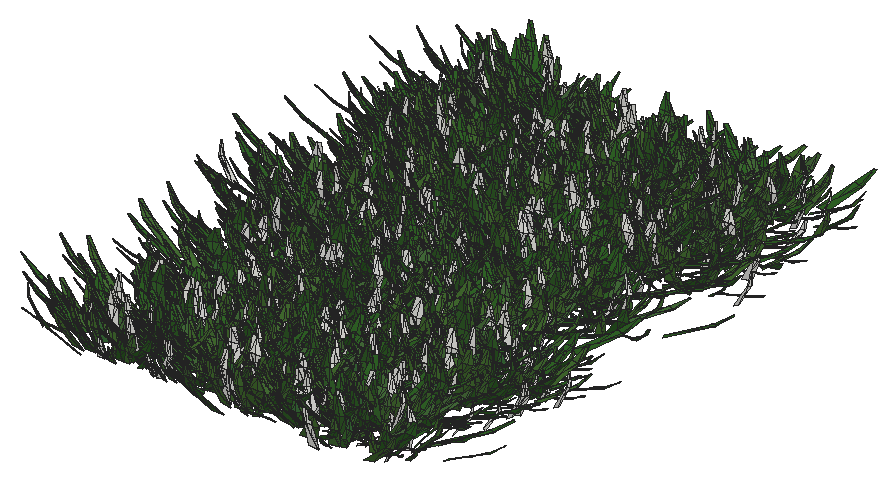
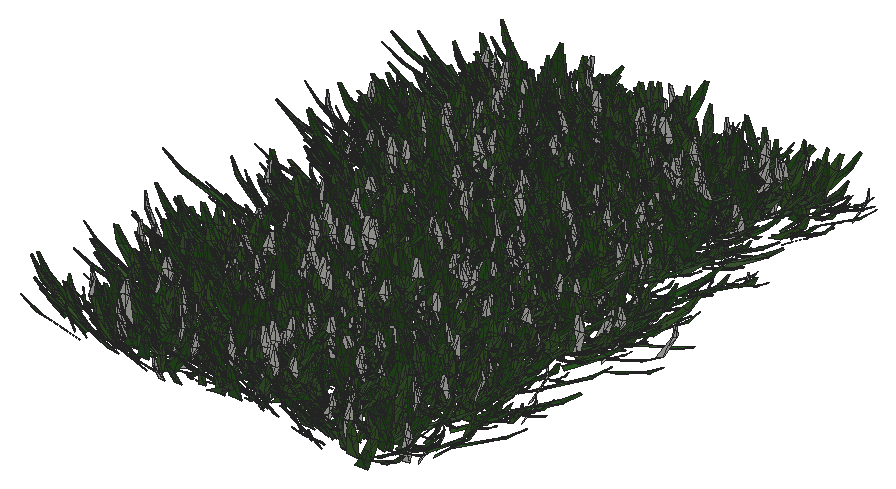
# SketchUp Ruby script. Lengths in inches.
U = 1.inch
M = Sketchup.active_model
def pt(a) = Geom::Point3d.new(a.map { |v| v * U })
def face(e, loops, mat)
  f = e.add_face(loops[0].map { |a| pt(a) })
  loops[1..].each { |l| e.add_face(l.map { |a| pt(a) }).erase! }
  f.material = f.back_material = mat if mat
  f
end
# faces: each face lists its corners as indices into pts; further lists are holes
def faces(e, pts, list, mat = nil) = list.each { |f| face(e, (f[0].is_a?(Array) ? f : [f]).map { |l| l.map { |i| pts[i] } }, mat) }
# xy, xz, yz: faces in a plane at the given z, y or x. An outline is a flat list of corners, or four numbers for a rectangle; further outlines are holes
def ring(l) = l.size == 4 ? [[l[0], l[1]], [l[2], l[1]], [l[2], l[3]], [l[0], l[3]]] : l.each_slice(2).to_a
def flat(e, list, mat, &to3) = list.each { |f| face(e, (f[0].is_a?(Array) ? f : [f]).map { |l| ring(l).map { |u, v| to3.(u, v) } }, mat) }
def xy(e, z, list, mat = nil) = flat(e, list, mat) { |x, y| [x, y, z] }
def xz(e, y, list, mat = nil) = flat(e, list, mat) { |x, z| [x, y, z] }
def yz(e, x, list, mat = nil) = flat(e, list, mat) { |y, z| [x, y, z] }
def lines(e, pts, list) = list.each { |a, b| e.add_line(pt(pts[a]), pt(pts[b])) }
# prism: a flat outline (further loops are holes) pulled along v
def prism(e, loops, v, mat = nil)
  f = face(e, loops, mat); d = Geom::Vector3d.new(v.map { |x| x * U })
  f.pushpull(f.normal.samedirection?(d) ? d.length : -d.length)
end
def box(e, o, s, mat = nil) = prism(e, [[o, [o[0] + s[0], o[1], o[2]], [o[0] + s[0], o[1] + s[1], o[2]], [o[0], o[1] + s[1], o[2]]]], [0, 0, s[2]], mat)
def at(x, y, z, deg = 0) = Geom::Transformation.translation(pt([x, y, z])) * Geom::Transformation.rotation(ORIGIN, Z_AXIS, deg.degrees)
def axes(o, x, y, z) = Geom::Transformation.new([*x, 0, *y, 0, *z, 0, *pt(o).to_a, 1])
def part(name) = M.definitions.add(name)
# library, detail: a bought-in or finely detailed component or shape, given as its bounding box
def library(name, o, s) = part(name).tap { |d| box(d.entities, o, s) }
def detail(e, o, s) = box(e.add_group.entities, o, s)
def put(e, d, t, mat = nil) = e.add_instance(d, t).tap { |i| i.material = mat if mat }
def group(e, t, mat = nil) = e.add_group.tap { |g| g.transformation = t; g.material = mat if mat }.entities
root = M.entities
M.materials.add("Material82").color = [68, 110, 58]
M.materials.add("Material83").color = [48, 90, 38]
M.materials.add("Material84").color = [68, 110, 48]
M.materials.add("Material85").color = [48, 90, 48]
M.materials.add("Material86").color = [58, 110, 58]
M.materials.add("Material87").color = [58, 90, 38]
M.materials.add("Material88").color = [68, 100, 58]
M.materials.add("Material89").color = [48, 100, 38]
c1 = part("grass00")
p = [[-0.6875,0.15,0],[-0.56,0.08,5.52],[-0.04,0.03,2.76],[0.48,-0.02,0],[0.35,-0.02,5.52],[-0.1,-0.14,5.52],
  [-0.12,0.65,8.37],[-0.42,0.65,8.37]]
faces(c1.entities,p,[[0,1,2,3],[3,2,4],[1,5,2],[5,4,2],[1,6,5],[4,5,6],[7,6,1]])
c2 = part("Group16\#1")
put(c2.entities,c1,axes([1.44,-0.61,-0.01],[0.05352,0.12609,0],[-0.10704,0.04543,0.07239],[0.06664,-0.02828,0.11628]),"Material85")
put(c2.entities,c1,axes([0.76,-0.15,-0.01],[0.04676,0.24062,0],[-0.23162,0.04501,0.06642],[0.0652,-0.01267,0.23595]),"Material82")
put(c2.entities,c1,axes([0.79,0.01,-0.01],[-0.00606,0.34651,0],[-0.34381,-0.00602,0.0432],[0.04319,0.00076,0.34386]))
put(c2.entities,c1,axes([1,0.23,-0.01],[-0.07192,0.31144,0],[-0.28722,-0.06632,0.1236],[0.12043,0.02781,0.29478]),"Material84")
put(c2.entities,c1,axes([1.66,0.77,-0.01],[-0.13828,0.29651,0],[-0.21551,-0.1005,0.22471],[0.20365,0.09498,0.23779]),"Material89")
put(c2.entities,c1,axes([0.6875,0.52,-0.01],[-0.18126,0.24051,0],[-0.22746,-0.17142,0.09788],[0.07817,0.05891,0.28481]),"Material84")
put(c2.entities,c1,axes([0.68,0.78,-0.01],[-0.215,0.18688,0],[-0.12385,-0.14248,0.21334],[0.13995,0.16101,0.18878]),"Material82")
put(c2.entities,c1,axes([0.56,1,-0.01],[-0.13756,0.07624,0],[-0.06159,-0.11112,0.0927],[0.04494,0.08108,0.12705]),"Material84")
put(c2.entities,c1,axes([0.2,0.64,-0.01],[-0.23729,0.07254,0],[-0.05711,-0.18681,0.153],[0.04473,0.14632,0.19535]),"Material89")
put(c2.entities,c1,axes([0.0625,0.72,-0.01],[-0.28874,0.02525,0],[-0.02179,-0.24916,0.14647],[0.01276,0.14591,0.25012]),"Material82")
put(c2.entities,c1,axes([-0.08,0.62,-0.01],[-0.34089,-0.04187,0],[0.03255,-0.26504,0.216],[-0.02633,0.21439,0.26703]),"Material89")
put(c2.entities,c1,axes([-0.34,0.98,-0.01],[-0.14314,-0.0493,0],[0.04397,-0.12769,0.06843],[-0.02228,0.0647,0.13505]),"Material89")
put(c2.entities,c1,axes([-0.87,1.45,-0.01],[-0.23488,-0.14114,0],[0.13761,-0.22901,0.06087],[-0.03135,0.05217,0.26717]))
put(c2.entities,c1,axes([-0.72,0.77,-0.01],[-0.14208,-0.13251,0],[0.07209,-0.0773,0.16301],[-0.11118,0.11922,0.1057]),"Material89")
put(c2.entities,c1,axes([-0.62,0.43,-0.01],[-0.14845,-0.21203,0],[0.18654,-0.13061,0.12304],[-0.10079,0.07057,0.22772]),"Material82")
put(c2.entities,c1,axes([-0.68,0.29,-0.01],[-0.13639,-0.32136,0],[0.31723,-0.13464,0.05579],[-0.05136,0.0218,0.34462]),"Material83")
put(c2.entities,c1,axes([-0.64,0.125,-0.01],[-0.0458,-0.23569,0],[0.22124,-0.043,0.08276],[-0.08124,0.01579,0.22538]),"Material86")
put(c2.entities,c1,axes([-1.6,-0.03,-0.01],[0.00576,-0.32897,0],[0.27526,0.00482,0.18018],[-0.18015,-0.00315,0.2753]),"Material84")
put(c2.entities,c1,axes([-1.36,-0.31,-0.01],[0.05718,-0.24765,0],[0.18172,0.04196,0.17267],[-0.16825,-0.03885,0.1865]),"Material89")
put(c2.entities,c1,axes([-1.54,-0.72,-0.01],[0.06537,-0.14017,0],[0.13555,0.06321,0.03939],[-0.0357,-0.01665,0.14956]))
put(c2.entities,c1,axes([-1.19,-0.9,-0.01],[0.09597,-0.12735,0],[0.11214,0.08451,0.07557],[-0.06035,-0.04548,0.14042]),"Material88")
put(c2.entities,c1,axes([-0.47,-0.54,-0.01],[0.11588,-0.10072,0],[0.0618,0.0711,0.12124],[-0.07953,-0.0915,0.0942]))
put(c2.entities,c1,axes([-0.47,-0.84,-0.01],[0.11927,-0.0661,0],[0.06603,0.11913,0.00646],[-0.00313,-0.00565,0.13621]),"Material84")
put(c2.entities,c1,axes([-0.38,-1.24,-0.01],[0.28037,-0.08571,0],[0.0618,0.20215,0.20315],[-0.05939,-0.19428,0.21139]),"Material88")
put(c2.entities,c1,axes([-0.06,-0.66,-0.01],[0.22719,-0.01987,0],[0.01247,0.14255,0.17758],[-0.01547,-0.17691,0.1431]),"Material87")
put(c2.entities,c1,axes([0.11,-0.89,-0.01],[0.14882,0.01828,0],[-0.01058,0.08611,0.12229],[0.01491,-0.12138,0.08676]),"Material85")
put(c2.entities,c1,axes([0.25,-0.72,-0.01],[0.20481,0.07053,0],[-0.06206,0.18022,0.10291],[0.03351,-0.0973,0.1906]),"Material85")
put(c2.entities,c1,axes([0.85,-1.42,-0.01],[0.16481,0.09904,0],[-0.09472,0.15762,0.05616],[0.02893,-0.04814,0.18389]),"Material84")
put(c2.entities,c1,axes([1.01,-1.09,-0.01],[0.21858,0.20385,0],[-0.17495,0.1876,0.15339],[0.10462,-0.11218,0.25652]),"Material89")
put(c2.entities,c1,axes([1.01,-0.71,-0.01],[0.08733,0.12473,0],[-0.06445,0.04512,0.13037],[0.1068,-0.07477,0.07867]),"Material85")
c3 = part("Group15\#1")
put(c3.entities,c2,at(0,0,0))
c4 = part("3darcstudiotree_grass00\#1")
put(c4.entities,c3,at(0,0,0))
put(root,c4,axes([1795.82,1028.89,-29.74],[-2.46131,1.0799,0],[-2.93079,-1.03891,-0.05045],[-0.18868,-0.06689,1.48531]))
put(root,c4,axes([1795.33,1042.55,-29.74],[0.6827,1.82438,0],[-3.27697,0.19072,-0.00575],[-0.03023,0.00176,1.31904]))
put(root,c4,axes([1795.52,997.3,-29.74],[0.45996,1.33665,0],[-3.57607,0.19139,-0.02967],[-0.17102,0.00915,1.57371]))
put(root,c4,axes([1797.45,1041.28,-29.74],[-3.10229,-1.16988,0],[2.93363,-1.20992,-0.00934],[0.03186,-0.01314,1.57129]))
put(root,c4,axes([1795.45,1024.93,-29.74],[2.66376,1.48543,0],[-3.56736,0.99495,-0.03132],[-0.13982,0.039,1.7905]))
put(root,c4,axes([1797.64,1044.75,-29.74],[-2.84959,-0.68183,0],[2.166,-1.40791,-0.04577],[0.14869,-0.09665,1.96036]))
put(root,c4,axes([1798.125,1042.05,-29.74],[-4.12072,-0.27119,0],[0.6549,-1.54771,-0.03361],[0.02858,-0.06755,1.54092]))
put(root,c4,axes([1798.11,996.66,-29.74],[-2.73846,-0.74739,0],[2.06192,-1.17502,-0.03348],[0.13147,-0.07492,1.87437]))
put(root,c4,axes([1798.46,1027.05,-29.74],[-1.65449,-1.67632,0],[3.5536,-0.54549,-0.00938],[0.04968,-0.00763,1.62403]))
put(root,c4,axes([1798.57,1016.8125,-29.74],[-2.10435,-1.3155,0],[3.64518,-0.9069,-0.04882],[0.17684,-0.044,1.38366]))
put(root,c4,axes([1798.44,1033.6,-29.74],[-3.62624,-0.35306,0],[1.02554,-1.63824,-0.03453],[0.0374,-0.05975,1.44935]))
put(root,c4,axes([1797.34,1039.09,-29.74],[0.82539,1.5958,0],[-3.41483,0.2747,-0.03877],[-0.28197,0.02268,1.93915]))
put(root,c4,axes([1797.72,1011.43,-29.74],[3.93831,-0.79818,0],[2.14355,1.64496,-0.04443],[0.08068,0.06192,1.39643]))
put(root,c4,axes([1798.98,1020.12,-29.74],[-2.03778,-1.0951,0],[3.7049,-1.07224,-0.05528],[0.23064,-0.06675,1.78248]))
put(root,c4,axes([1799,1019.15,-29.74],[-3.67688,-0.6634,0],[1.45076,-1.25058,-0.02741],[0.08145,-0.07021,1.86713]))
put(root,c4,axes([1797.36,1023.27,-29.74],[3.8654,0.35733,0],[-0.81256,1.36706,-0.007],[-0.00937,0.01576,1.56436]))
put(root,c4,axes([1797.62,1029.81,-29.74],[0.38941,1.44392,0],[-4.06327,0.17043,-0.05804],[-0.26328,0.01104,1.39706]))
put(root,c4,axes([1797.61,1050.98,-29.74],[3.44355,0.26807,0],[-0.70938,1.41724,-0.02055],[-0.0272,0.05435,1.87683]))
put(root,c4,axes([1799.38,1007.75,-29.74],[-3.021,-0.6477,0],[1.60996,-1.16789,-0.02167],[0.0547,-0.03968,1.33527]))
put(root,c4,axes([1799.25,1036.58,-29.74],[-4.07234,0.0884,0],[-0.21728,-1.55677,-0.00024],[-0.00008,-0.0006,1.85086]))
put(root,c4,axes([1798.98,999.31,-29.74],[-3.52536,0.66718,0],[-1.57507,-1.29441,-0.02803],[-0.08559,-0.07034,1.92571]))
put(root,c4,axes([1798.1,1053.3125,-29.74],[0.25287,1.52902,0],[-3.62555,0.09325,-0.03468],[-0.21891,0.00563,1.72254]))
put(root,c4,axes([1798.55,1014.4375,-29.74],[3.86172,-0.56351,0],[1.21864,1.29888,-0.04569],[0.10723,0.11428,1.78027]))
put(root,c4,axes([1799.83,1049.22,-29.74],[-4.49885,0.1512,0],[-0.3136,-1.45126,-0.04489],[-0.02566,-0.11876,1.86365]))
put(root,c4,axes([1799.33,1009.58,-29.74],[2.47969,-0.8558,0],[2.79846,1.26111,-0.0129],[0.03707,0.01671,1.39029]))
put(root,c4,axes([1799.05,1025.95,-29.74],[3.77184,-0.74152,0],[2.04611,1.61872,-0.00236],[0.0043,0.00341,1.40454]))
put(root,c4,axes([1800.25,1047.68,-29.74],[-3.95195,-0.11479,0],[0.31612,-1.69258,-0.00991],[0.00383,-0.02049,1.69565]))
put(root,c4,axes([1799,1003.09,-29.74],[4.4523,-0.10128,0],[0.21715,1.4846,-0.03809],[0.01394,0.09529,1.79573]))
put(root,c4,axes([1799.4375,1001.68,-29.74],[3.96943,-0.89247,0],[1.86138,1.2876,-0.05304],[0.17378,0.12021,1.86337]))
put(root,c4,axes([1800.85,1005.29,-29.74],[-0.06079,-1.40056,0],[3.30003,-0.02228,-0.01279],[0.0855,-0.00058,1.65408]))
put(root,c4,axes([1800.79,1031.88,-29.74],[-0.47592,1.56401,0],[-3.26389,-0.15447,-0.01529],[-0.10295,-0.00487,1.67142]))
put(root,c4,axes([1802.8,1006.18,-29.74],[-0.30634,-1.35211,0],[4.22133,-0.14875,-0.01785],[0.10663,-0.00376,1.90542]))
put(root,c4,axes([1802.88,1006.96,-29.74],[0.00917,-1.7323,0],[3.83355,0.00316,-0.00952],[0.04811,0.00004,1.45276]))
put(root,c4,axes([1803.4,1031.06,-29.74],[-3.94041,-0.17555,0],[0.52244,-1.82386,-0.03054],[0.01805,-0.06303,1.83699]))
put(root,c4,axes([1803.51,1038.49,-29.74],[-3.62534,0.37466,0],[-0.93047,-1.40031,-0.00505],[-0.0081,-0.01218,1.74136]))
put(root,c4,axes([1802.82,1022.87,-29.74],[3.51422,-0.54071,0],[1.19989,1.21289,-0.03886],[0.08676,0.0877,1.52001]))
put(root,c4,axes([1804.48,1051.37,-29.74],[-3.51186,-0.721,0],[1.80955,-1.37083,-0.02288],[0.05511,-0.04175,1.53217]))
put(root,c4,axes([1804.5,1029.875,-29.74],[1.44921,-1.37247,0],[3.47001,0.56986,-0.04485],[0.23379,0.03839,1.59096]))
put(root,c4,axes([1803.62,1002.98,-29.74],[0.66388,1.42145,0],[-3.998,0.29041,-0.0472],[-0.22325,0.01622,1.46547]))
put(root,c4,axes([1803.72,1025.51,-29.74],[2.60904,1.49403,0],[-2.88542,0.78369,-0.04649],[-0.18984,0.05156,1.30192]))
put(root,c4,axes([1803.84,1013.72,-29.74],[3.83063,0.28141,0],[-0.63066,1.33518,-0.03922],[-0.04064,0.08605,1.46066]))
put(root,c4,axes([1804.38,1028.07,-29.74],[2.98326,-0.56932,0],[1.56375,1.27443,-0.0104],[0.02417,0.0197,1.43546]))
put(root,c4,axes([1803.78,1039.72,-29.74],[0.44153,1.60869,0],[-4.59886,0.19631,-0.03135],[-0.13775,0.00588,1.53244]))
put(root,c4,axes([1804.41,1042.45,-29.74],[3.7963,-0.32727,0],[0.82791,1.49367,-0.02018],[0.02229,0.04022,1.50307]))
put(root,c4,axes([1806.37,1018.1,-29.74],[-2.44222,-1.21448,0],[3.27109,-1.02306,-0.01126],[0.03735,-0.01168,1.32461]))
put(root,c4,axes([1806.04,1012.8,-29.74],[-3.39135,-0.3159,0],[0.83318,-1.39116,-0.01801],[0.02035,-0.03397,1.33554]))
put(root,c4,axes([1805.92,1009.53,-29.74],[-1.25644,-1.35671,0],[3.16457,-0.45581,-0.03784],[0.23357,-0.03364,1.65933]))
put(root,c4,axes([1806.32,1046.6,-29.74],[-0.2827,-1.72948,0],[4.63241,-0.11777,-0.03565],[0.15653,-0.00398,1.53082]))
put(root,c4,axes([1806.47,1020.64,-29.74],[-4.6912,-0.24024,0],[0.57575,-1.74859,-0.02421],[0.01544,-0.0469,1.66024]))
put(root,c4,axes([1805.57,1045.24,-29.74],[2.39093,-1.03283,0],[3.02488,1.08907,-0.05494],[0.24262,0.08735,1.83588]))
put(root,c4,axes([1805.59,1001.06,-29.74],[3.97766,0.18345,0],[-0.40911,1.37962,-0.0104],[-0.00856,0.02886,1.87036]))
put(root,c4,axes([1806.44,1036.82,-29.74],[2.63553,-1.14097,0],[3.49929,1.25715,-0.04921],[0.17097,0.06142,1.66765]))
put(root,c4,axes([1806.3125,1034.22,-29.74],[-2.26024,1.36544,0],[-3.77789,-0.97262,-0.02867],[-0.12669,-0.03262,1.78429]))
put(root,c4,axes([1805.84,997.26,-29.74],[2.88281,0.64392,0],[-1.76321,1.22772,-0.02459],[-0.08623,0.06004,1.90817]))
put(root,c4,axes([1806.53,1016.9375,-29.74],[3.80429,-0.95187,0],[2.21902,1.37934,-0.04672],[0.14892,0.09257,1.84728]))
put(root,c4,axes([1805.92,998.35,-29.74],[3.38308,1.28097,0],[-3.13031,1.28579,-0.04664],[-0.1697,0.06971,1.77978]))
put(root,c4,axes([1806.52,1048.77,-29.74],[1.17272,1.70605,0],[-3.75992,0.40197,-0.02312],[-0.1149,0.01228,1.50331]))
put(root,c4,axes([1808.88,1020.29,-29.74],[2.08515,-1.11593,0],[3.14779,0.91479,-0.04551],[0.20545,0.05971,1.64335]))
put(root,c4,axes([1808.92,1014.2,-29.74],[-2.84594,1.17329,0],[-3.06349,-1.15571,-0.01205],[-0.05136,-0.01938,1.87482]))
put(root,c4,axes([1809.95,1004.18,-29.74],[-4.1718,-0.04402,0],[0.1133,-1.66995,-0.01377],[0.00192,-0.02825,1.65227]))
put(root,c4,axes([1809.53,1028.09,-29.74],[-3.19418,0.83767,0],[-2.09756,-1.24397,-0.00165],[-0.00457,-0.00271,1.42237]))
put(root,c4,axes([1810.47,1009.56,-29.74],[-3.23677,-0.61439,0],[2.0349,-1.66734,-0.00367],[0.00726,-0.00595,1.60507]))
put(root,c4,axes([1810.08,1001.03,-29.74],[0.66157,-1.84804,0],[3.88634,0.21638,-0.01886],[0.11067,0.00616,1.74385]))
put(root,c4,axes([1809.09,1024.71,-29.74],[3.70848,0.20038,0],[-0.48617,1.3994,-0.00884],[-0.00845,0.02433,1.89082]))
put(root,c4,axes([1809.24,1049.92,-29.74],[3.47876,0.69717,0],[-2.07434,1.60981,-0.02666],[-0.05222,0.04053,1.48409]))
put(root,c4,axes([1809.8,998.35,-29.74],[-1.68767,1.14523,0],[-4.10192,-0.94014,-0.02835],[-0.11929,-0.02734,1.73088]))
put(root,c4,axes([1811.25,1042.89,-29.74],[-4.10821,-0.63147,0],[1.40621,-1.42285,-0.03755],[0.0732,-0.07407,1.55797]))
put(root,c4,axes([1809.81,1039.9,-29.74],[4.36048,0.20882,0],[-0.42656,1.38529,-0.01966],[-0.01597,0.05186,1.78732]))
put(root,c4,axes([1810.25,1031.31,-29.74],[-1.75851,1.2095,0],[-3.69968,-0.83659,-0.01882],[-0.09945,-0.02249,1.94745]))
put(root,c4,axes([1811.78,1038.96,-29.74],[-1.44336,-1.26835,0],[3.91991,-0.69378,-0.01184],[0.05292,-0.00937,1.57815]))
put(root,c4,axes([1811.55,1044.71,-29.74],[-0.45128,-1.33361,0],[4.22591,-0.22241,-0.03174],[0.17504,-0.00921,1.77768]))
put(root,c4,axes([1810.6,1007.53,-29.74],[3.82795,-0.89848,0],[2.12017,1.40489,-0.02674],[0.0662,0.04387,1.50406]))
put(root,c4,axes([1811.68,1047.18,-29.74],[-2.48368,-1.57939,0],[3.38438,-0.82775,-0.05324],[0.27998,-0.06848,1.84703]))
put(root,c4,axes([1811.55,1022.47,-29.74],[-3.70161,0.1835,0],[-0.55617,-1.74492,-0.04842],[-0.0352,-0.11043,1.94818]))
put(root,c4,axes([1812.1,996.95,-29.74],[-2.02199,-1.57321,0],[3.0284,-0.60536,-0.03791],[0.25064,-0.0501,1.88609]))
put(root,c4,axes([1810.75,1019.16,-29.74],[4.60425,0.18746,0],[-0.4763,1.81947,-0.06196],[-0.02818,0.10763,1.53928]))
put(root,c4,axes([1810.97,1005.1,-29.74],[3.66376,0.25232,0],[-0.75626,1.7079,-0.04039],[-0.02947,0.06656,1.39779]))
put(root,c4,axes([1811.21,1016.97,-29.74],[3.38223,0.96892,0],[-2.45655,1.33368,-0.05492],[-0.16887,0.09168,1.63919]))
put(root,c4,axes([1812.4,1050.81,-29.74],[-3.51929,1.02852,0],[-2.47816,-1.3188,-0.03727],[-0.13373,-0.07117,1.88005]))
put(root,c4,axes([1811.85,1030.35,-29.74],[3.59827,-1.20315,0],[2.55541,1.18863,-0.04452],[0.1901,0.08842,1.95574]))
put(root,c4,axes([1811.0625,1034.56,-29.74],[2.55345,1.05656,0],[-3.3838,1.27189,-0.0237],[-0.06613,0.02486,1.35093]))
put(root,c4,axes([1812.11,1012.71,-29.74],[3.17823,1.19717,0],[-2.46254,1.01678,-0.00574],[-0.02103,0.00868,1.41814]))
put(root,c4,axes([1812.3125,1036.57,-29.74],[1.4209,1.26091,0],[-3.92098,0.6872,-0.00487],[-0.02309,0.00405,1.66894]))
put(root,c4,axes([1814.98,1001.15,-29.74],[-4.20115,-0.27572,0],[0.6063,-1.43684,-0.03971],[0.03476,-0.08238,1.4765]))
put(root,c4,axes([1814.32,1047.37,-29.74],[-2.56197,0.85481,0],[-2.91428,-1.35846,-0.04396],[-0.15305,-0.07134,1.82298]))
put(root,c4,axes([1814.39,1048.45,-29.74],[-3.07207,1.32257,0],[-2.98229,-1.07739,-0.02313],[-0.10886,-0.03933,1.93523]))
put(root,c4,axes([1814.39,1007.88,-29.74],[3.03154,-1.30842,0],[2.70015,0.973,-0.04297],[0.17128,0.06172,1.48019]))
put(root,c4,axes([1814.29,1010.51,-29.74],[4.0708,-0.43574,0],[1.12817,1.63922,-0.0215],[0.0298,0.0433,1.70776]))
put(root,c4,axes([1814.06,1035.875,-29.74],[1.45585,1.40356,0],[-4.29762,0.69331,-0.06498],[-0.33385,0.05386,1.93183]))
put(root,c4,axes([1814.62,1021.4,-29.74],[3.98961,-0.74286,0],[1.49364,1.24762,-0.01833],[0.03992,0.03334,1.33779]))
put(root,c4,axes([1814.54,1023.45,-29.74],[-1.90909,1.29111,0],[-3.77719,-0.86865,-0.00159],[-0.00678,-0.00156,1.61385]))
put(root,c4,axes([1814.47,1042.29,-29.74],[3.44974,0.13102,0],[-0.35474,1.45265,-0.03978],[-0.02715,0.11118,1.9745]))
put(root,c4,axes([1815.1,1031.26,-29.74],[4.01141,-0.57098,0],[1.38004,1.50792,-0.00463],[0.00922,0.01007,1.7876]))
put(root,c4,axes([1816.61,999.71,-29.74],[-2.56515,-0.8375,0],[2.7288,-1.2999,-0.02106],[0.06081,-0.02897,1.45262]))
put(root,c4,axes([1814.59,1017.93,-29.74],[1.21271,1.28553,0],[-4.16441,0.61099,-0.01219],[-0.04469,0.00656,1.30286]))
put(root,c4,axes([1815.83,1011.61,-29.74],[-3.04036,1.06501,0],[-2.34315,-1.04035,-0.02123],[-0.07304,-0.03243,1.37003]))
put(root,c4,axes([1816.04,1017.28,-29.74],[1.27723,-1.67859,0],[3.60633,0.42678,-0.0465],[0.22987,0.0272,1.45674]))
put(root,c4,axes([1815.11,1005.15,-29.74],[4.09443,-0.06366,0],[0.15428,1.54325,-0.03451],[0.00867,0.0867,1.8714]))
put(root,c4,axes([1816.88,1051.75,-29.74],[-2.71598,-1.39793,0],[3.51357,-1.0617,-0.04805],[0.18587,-0.05616,1.61679]))
put(root,c4,axes([1815.06,1003.16,-29.74],[3.43879,0.48398,0],[-1.47194,1.62658,-0.03925],[-0.05225,0.05774,1.29995]))
put(root,c4,axes([1816.44,1044.11,-29.74],[0.94515,-1.66762,0],[4.07339,0.35906,-0.0396],[0.18346,0.01617,1.48525]))
put(root,c4,axes([1815.98,1034.39,-29.74],[2.86215,-0.69885,0],[2.15737,1.37418,-0.03178],[0.09016,0.05743,1.65559]))
put(root,c4,axes([1815.7,1039.95,-29.74],[2.07536,1.00802,0],[-2.97078,0.95128,-0.04172],[-0.20153,0.06453,1.78477]))
put(root,c4,axes([1817.24,1037.93,-29.74],[0.03648,-1.32003,0],[3.51668,0.01511,-0.01263],[0.08154,0.00035,1.70174]))
put(root,c4,axes([1817.47,1013.93,-29.74],[-0.06785,-1.57512,0],[4.70678,-0.03153,-0.0635],[0.34719,-0.00233,1.92948]))
put(root,c4,axes([1817.1,1027.73,-29.74],[-0.80195,1.7338,0],[-4.65742,-0.33505,-0.02378],[-0.12913,-0.00929,1.95907]))
put(root,c4,axes([1817.41,997.23,-29.74],[-1.48177,1.26839,0],[-3.97677,-0.72256,-0.00587],[-0.02393,-0.00435,1.47291]))
put(root,c4,axes([1817.44,1028.88,-29.74],[4.46941,0.03034,0],[-0.07094,1.62545,-0.04862],[-0.00377,0.08633,1.39123]))
put(root,c4,axes([1817.92,1024.98,-29.74],[3.5964,-0.66598,0],[1.43149,1.20228,-0.03796],[0.09777,0.08212,1.52986]))
put(root,c4,axes([1819.86,1007.8,-29.74],[-3.83088,0.01586,0],[-0.04003,-1.50367,-0.01485],[-0.00089,-0.03334,1.62647]))
put(root,c4,axes([1819.75,1036.53,-29.74],[2.50638,-0.90958,0],[2.96207,1.26944,-0.00074],[0.00258,0.00111,1.68668]))
put(root,c4,axes([1820.36,1021.55,-29.74],[-1.26463,-1.25515,0],[3.81596,-0.59798,-0.04918],[0.19961,-0.03128,1.34418]))
put(root,c4,axes([1819.8,1029.59,-29.74],[-2.59269,1.36416,0],[-3.43206,-1.0145,-0.01976],[-0.08545,-0.02526,1.7373]))
put(root,c4,axes([1819.56,1031.63,-29.74],[4.23995,-0.14734,0],[0.39715,1.77755,-0.00682],[0.00263,0.01179,1.49182]))
put(root,c4,axes([1820.81,1023.46,-29.74],[0.54946,-1.30633,0],[4.42126,0.28923,-0.06063],[0.27406,0.01793,1.53907]))
put(root,c4,axes([1819.66,1045.02,-29.74],[4.19345,0.64908,0],[-1.43857,1.4455,-0.00074],[-0.00143,0.00144,1.56313]))
put(root,c4,axes([1821.63,1033.59,-29.74],[-4.00947,-0.30727,0],[0.87061,-1.76683,-0.00093],[0.00074,-0.0015,1.42207]))
put(root,c4,axes([1821.76,1042.25,-29.74],[-2.04014,-1.04561,0],[3.14641,-0.95481,-0.03027],[0.11908,-0.03613,1.47708]))
put(root,c4,axes([1820.01,1027.68,-29.74],[0.66214,1.69294,0],[-3.60919,0.21955,-0.0058],[-0.03794,0.00231,1.813]))
put(root,c4,axes([1821.26,996.64,-29.74],[-3.15684,0.83052,0],[-1.94414,-1.14932,-0.03251],[-0.12313,-0.07279,1.79208]))
put(root,c4,axes([1821.5,1011.55,-29.74],[1.45773,-1.41559,0],[3.72691,0.5969,-0.04502],[0.25742,0.04123,1.86083]))
put(root,c4,axes([1821.17,1001.95,-29.74],[3.14963,-1.20842,0],[2.29792,0.93151,-0.01443],[0.07601,0.03081,1.86565]))
put(root,c4,axes([1822.33,1015.89,-29.74],[-4.00454,-0.52801,0],[1.05814,-1.24816,-0.00172],[0.00311,-0.00367,1.42531]))
put(root,c4,axes([1822.43,1002.76,-29.74],[-1.0046,-1.54951,0],[3.94346,-0.39764,-0.04783],[0.24428,-0.02463,1.6084]))
put(root,c4,axes([1822.75,1040.2,-29.74],[-2.23262,-1.3088,0],[3.58665,-0.95157,-0.0439],[0.1738,-0.04611,1.54604]))
put(root,c4,axes([1820.93,1025.83,-29.74],[2.75664,0.78459,0],[-2.60411,1.42301,-0.01696],[-0.0547,0.02989,1.8379]))
put(root,c4,axes([1821.15,1015.01,-29.74],[1.57656,1.15501,0],[-3.7913,0.80487,-0.00648],[-0.02974,0.00631,1.68262]))
put(root,c4,axes([1822.96,1051.72,-29.74],[-4.26955,0.05297,0],[-0.11438,-1.43394,-0.03177],[-0.00727,-0.09116,1.98473]))
put(root,c4,axes([1821.35,1046.57,-29.74],[3.41924,1.14131,0],[-2.67356,1.24575,-0.04954],[-0.1842,0.08583,1.78537]))
put(root,c4,axes([1823.45,1004.75,-29.74],[-0.37683,-1.42813,0],[4.6236,-0.18974,-0.00351],[0.01488,-0.00061,1.48465]))
put(root,c4,axes([1821.65,999.82,-29.74],[4.54007,0.12562,0],[-0.30482,1.71344,-0.05051],[-0.02069,0.11631,1.91076]))
put(root,c4,axes([1823.45,1049.48,-29.74],[-2.30012,-1.16982,0],[2.63485,-0.80575,-0.0081],[0.04804,-0.01469,1.87526]))
put(root,c4,axes([1823.09,1038.24,-29.74],[0.45602,-1.75469,0],[4.51141,0.18235,-0.06373],[0.28019,0.01133,1.50237]))
put(root,c4,axes([1823.05,1009.14,-29.74],[1.62707,-1.18617,0],[3.8873,0.82932,-0.03985],[0.15889,0.0339,1.5017]))
put(root,c4,axes([1822.61,1018.41,-29.74],[4.17569,0.70475,0],[-1.86329,1.71705,-0.06274],[-0.13365,0.12316,1.92197]))
put(root,c4,axes([1825.02,1010.7,-29.74],[-3.80347,-0.79702,0],[1.88494,-1.39901,-0.03648],[0.10192,-0.07565,1.79293]))
put(root,c4,axes([1824.95,1008.4,-29.74],[-2.17021,-1.46243,0],[2.84473,-0.65657,-0.0221],[0.14072,-0.03248,1.82262]))
put(root,c4,axes([1824.99,999.1,-29.74],[3.21046,-0.42194,0],[1.31397,1.55496,-0.01535],[0.02427,0.02872,1.5577]))
put(root,c4,axes([1826.28,1040.96,-29.74],[-3.29126,-0.79109,0],[1.80045,-1.16502,-0.03312],[0.11366,-0.07354,1.70984]))
put(root,c4,axes([1825.97,1044.58,-29.74],[0.99321,-1.58581,0],[3.96504,0.38623,-0.04714],[0.20087,0.01957,1.34372]))
put(root,c4,axes([1826.52,1012.83,-29.74],[-2.18591,-1.17845,0],[3.11783,-0.89946,-0.02018],[0.10185,-0.02938,1.81061]))
put(root,c4,axes([1825.21,1026.88,-29.74],[4.09864,-0.14348,0],[0.37168,1.65134,-0.01913],[0.00999,0.04439,1.86132]))
put(root,c4,axes([1826.91,1036.55,-29.74],[-2.13357,-1.0721,0],[3.45076,-1.06807,-0.04646],[0.2021,-0.06255,1.81816]))
put(root,c4,axes([1825.08,1050.68,-29.74],[3.51961,1.01739,0],[-2.56437,1.37974,-0.04132],[-0.14142,0.07609,1.88254]))
put(root,c4,axes([1825.82,1014.65,-29.74],[-1.78032,1.61918,0],[-3.86174,-0.66038,-0.00354],[-0.01693,-0.0029,1.64409]))
